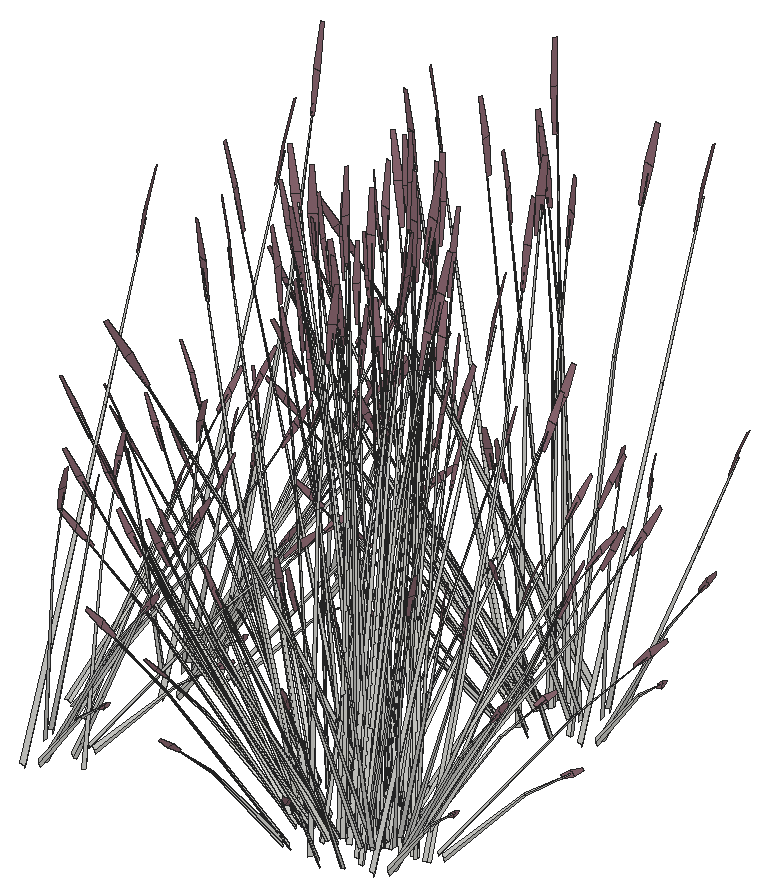
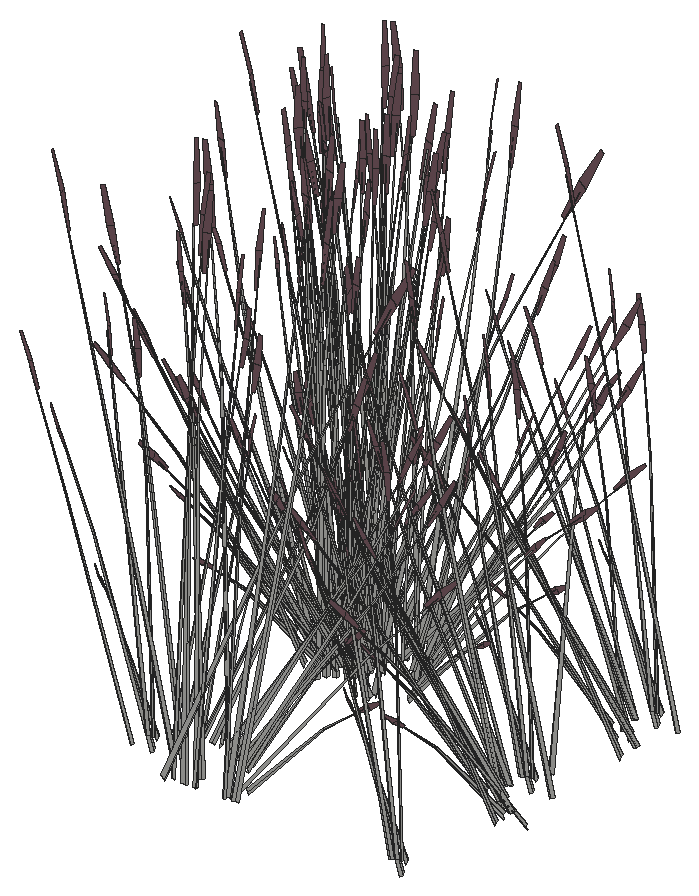
# SketchUp Ruby script. Lengths in inches.
U = 1.inch
M = Sketchup.active_model
def pt(a) = Geom::Point3d.new(a.map { |v| v * U })
def face(e, loops, mat)
  f = e.add_face(loops[0].map { |a| pt(a) })
  loops[1..].each { |l| e.add_face(l.map { |a| pt(a) }).erase! }
  f.material = f.back_material = mat if mat
  f
end
# faces: each face lists its corners as indices into pts; further lists are holes
def faces(e, pts, list, mat = nil) = list.each { |f| face(e, (f[0].is_a?(Array) ? f : [f]).map { |l| l.map { |i| pts[i] } }, mat) }
# xy, xz, yz: faces in a plane at the given z, y or x. An outline is a flat list of corners, or four numbers for a rectangle; further outlines are holes
def ring(l) = l.size == 4 ? [[l[0], l[1]], [l[2], l[1]], [l[2], l[3]], [l[0], l[3]]] : l.each_slice(2).to_a
def flat(e, list, mat, &to3) = list.each { |f| face(e, (f[0].is_a?(Array) ? f : [f]).map { |l| ring(l).map { |u, v| to3.(u, v) } }, mat) }
def xy(e, z, list, mat = nil) = flat(e, list, mat) { |x, y| [x, y, z] }
def xz(e, y, list, mat = nil) = flat(e, list, mat) { |x, z| [x, y, z] }
def yz(e, x, list, mat = nil) = flat(e, list, mat) { |y, z| [x, y, z] }
def lines(e, pts, list) = list.each { |a, b| e.add_line(pt(pts[a]), pt(pts[b])) }
# prism: a flat outline (further loops are holes) pulled along v
def prism(e, loops, v, mat = nil)
  f = face(e, loops, mat); d = Geom::Vector3d.new(v.map { |x| x * U })
  f.pushpull(f.normal.samedirection?(d) ? d.length : -d.length)
end
def box(e, o, s, mat = nil) = prism(e, [[o, [o[0] + s[0], o[1], o[2]], [o[0] + s[0], o[1] + s[1], o[2]], [o[0], o[1] + s[1], o[2]]]], [0, 0, s[2]], mat)
def at(x, y, z, deg = 0) = Geom::Transformation.translation(pt([x, y, z])) * Geom::Transformation.rotation(ORIGIN, Z_AXIS, deg.degrees)
def axes(o, x, y, z) = Geom::Transformation.new([*x, 0, *y, 0, *z, 0, *pt(o).to_a, 1])
def part(name) = M.definitions.add(name)
# library, detail: a bought-in or finely detailed component or shape, given as its bounding box
def library(name, o, s) = part(name).tap { |d| box(d.entities, o, s) }
def detail(e, o, s) = box(e.add_group.entities, o, s)
def put(e, d, t, mat = nil) = e.add_instance(d, t).tap { |i| i.material = mat if mat }
def group(e, t, mat = nil) = e.add_group.tap { |g| g.transformation = t; g.material = mat if mat }.entities
root = M.entities
M.materials.add("LightPink_Translucent").color = [144, 107, 117]
c1 = part("blade")
p = [[2.15,0.21,22],[0,0.17,0],[0.09,0.45,0],[2.18,0.31,22],[2.29,0.31,22],[0.38,0.45,0],
  [2.48,0.24,33],[2.49,0.24,33],[2.48,0.22,33]]
faces(c1.entities,p,[[0,1,2,3],[4,5,2,3],[6,3,4,7],[8,0,3,6]])
c2 = part("seeds")
p = [[0.3,-0.1,1.38],[-0.01,-0.03,1.59],[-0.01,-0.03,0.03],[0.14,-0.07,-0.07],[0.29,-0.03,3],[0.15,0.01,3.11]]
faces(c2.entities,p,[[0,1,2,3],[1,0,4,5]],"LightPink_Translucent")
c3 = part("blade with seeds")
put(c3.entities,c1,at(0,0,0))
put(c3.entities,c2,axes([2.4,0.25,30.99],[1.5799,-0.05474,1.17369],[-0.12525,1.92788,0.29478],[-0.07173,-0.02425,1.56792]))
put(root,c3,axes([34.53,26.82,44.92],[-0.78586,-0.03248,1.0506],[0.51898,-0.68985,0.58006],[0.31045,0.24509,0.8241]))
put(root,c3,axes([35.76,34.52,46.53],[0.82919,-0.54528,-0.35414],[0.78493,0.62262,0.4572],[0.11943,-0.31634,0.87481]))
put(root,c3,axes([35.96,41.53,44.77],[-0.69001,-0.29779,1.1486],[0.89096,-0.30257,0.84392],[0.24031,0.2563,0.25299]))
put(root,c3,axes([33.51,41.21,44.59],[0.02163,-0.34331,1.43002],[1.03345,-0.38348,-0.30754],[0.31903,0.4109,0.61141]))
put(root,c3,axes([38.05,38.59,44.375],[1.53239,0,0],[0,1.1575,-0.51607],[0,0.26363,1.63711]))
put(root,c3,axes([32.86,25.875,46.93],[1.20928,-0.24619,-0.51099],[0.21154,0.93233,-0.3958],[0.32481,0.26718,0.97773]))
put(root,c3,axes([33.97,18.58,44.63],[0.7662,-1.03778,0],[1.28187,0.57875,-0.51607],[0.29196,0.13181,1.63711]))
put(root,c3,axes([36.07,42.88,44.67],[-0.78586,-0.03248,1.0506],[0.51898,-0.68985,0.58006],[0.31045,0.24509,0.8241]))
put(root,c3,axes([35.22,20.32,46.93],[-0.31482,-0.94565,-0.51099],[1.19224,-0.16542,-0.3958],[0.34166,-0.254,0.97773]))
put(root,c3,axes([38.42,21.8,44.51],[-0.75977,-0.66224,-0.06488],[0.83212,-0.6068,-0.29416],[0.23578,-0.04272,0.97024]))
put(root,c3,axes([34.4,41.9375,46.68],[1.20928,-0.24619,-0.51099],[0.21154,0.93233,-0.3958],[0.32481,0.26718,0.97773]))
put(root,c3,axes([36.68,18.43,45.02],[-0.40819,0.5272,1.1486],[-0.35086,-0.70831,0.84392],[0.33713,-0.17749,0.25299]))
put(root,c3,axes([35.51,34.64,44.375],[0.7662,-1.03778,0],[1.28187,0.57875,-0.51607],[0.29196,0.13181,1.63711]))
put(root,c3,axes([36.46,55.41,46.68],[-0.31482,-0.94565,-0.51099],[1.19224,-0.16542,-0.3958],[0.34166,-0.254,0.97773]))
put(root,c3,axes([36.76,36.375,46.68],[-0.31482,-0.94565,-0.51099],[1.19224,-0.16542,-0.3958],[0.34166,-0.254,0.97773]))
put(root,c3,axes([35.25,20.7,47.23],[0.64013,-0.81717,-0.71045],[1.12174,0.58074,0.08574],[0.38221,-0.29607,1.00501]))
put(root,c3,axes([37.93,53.52,44.77],[-0.40819,0.5272,1.1486],[-0.35086,-0.70831,0.84392],[0.33713,-0.17749,0.25299]))
put(root,c3,axes([38.22,34.49,44.77],[-0.40819,0.5272,1.1486],[-0.35086,-0.70831,0.84392],[0.33713,-0.17749,0.25299]))
put(root,c3,axes([37.34,55.5,46.53],[1.06674,-0.14801,-0.35414],[0.28168,0.84611,0.4572],[0.30569,-0.22726,0.87481]))
put(root,c3,axes([36.49,55.79,46.98],[0.64013,-0.81717,-0.71045],[1.12174,0.58074,0.08574],[0.38221,-0.29607,1.00501]))
put(root,c3,axes([37.64,36.48,46.53],[1.06674,-0.14801,-0.35414],[0.28168,0.84611,0.4572],[0.30569,-0.22726,0.87481]))
put(root,c3,axes([35.77,22.42,46.93],[0.332,-0.94205,-0.51099],[1.13828,0.3229,-0.3958],[0.45829,-0.08638,0.97773]))
put(root,c3,axes([36.79,36.76,46.98],[0.64013,-0.81717,-0.71045],[1.12174,0.58074,0.08574],[0.38221,-0.29607,1.00501]))
put(root,c3,axes([38.63,23.02,45.02],[-0.75718,0.17097,1.1486],[0.35641,-0.70661,0.84392],[0.40168,0.04835,0.25299]))
put(root,c3,axes([36.78,41.16,46.53],[0.69728,0.64842,-0.35414],[-0.79619,0.61382,0.4572],[0.40453,0.09339,0.87481]))
put(root,c3,axes([36.17,19.95,44.84],[-0.4378,-0.03068,1.43002],[-0.44851,-0.8229,-0.30754],[0.53783,-0.23279,0.61141]))
put(root,c3,axes([34.5,24.66,47.23],[1.22504,0.02494,-0.71045],[-0.08228,1.05005,0.08574],[0.51899,0.11081,1.00501]))
put(root,c3,axes([36.99,22.68,44.23],[-0.7893,0.12429,1.41583],[-0.12563,-0.9893,0.08104],[0.55282,-0.14974,0.80566]))
put(root,c3,axes([37.3125,38.48,46.68],[0.332,-0.94205,-0.51099],[1.13828,0.3229,-0.3958],[0.45829,-0.08638,0.97773]))
put(root,c3,axes([40.17,39.08,44.77],[-0.75718,0.17097,1.1486],[0.35641,-0.70661,0.84392],[0.40168,0.04835,0.25299]))
put(root,c3,axes([37.42,55.04,44.59],[-0.4378,-0.03068,1.43002],[-0.44851,-0.8229,-0.30754],[0.53783,-0.23279,0.61141]))
put(root,c3,axes([35.55,22.76,47.23],[1.07686,-0.45739,-0.71045],[0.60013,0.94154,0.08574],[0.52031,-0.10696,1.00501]))
put(root,c3,axes([37.72,36.01,44.59],[-0.4378,-0.03068,1.43002],[-0.44851,-0.8229,-0.30754],[0.53783,-0.23279,0.61141]))
put(root,c3,axes([38.01,38.91,46.53],[1.01846,0.28891,-0.35414],[-0.29705,0.84289,0.4572],[0.41005,-0.07729,0.87481]))
put(root,c3,axes([56.85,28.2,44.59],[0.42589,0.08502,1.43002],[0.2745,0.86839,-0.30754],[-0.57851,0.16255,0.61141]))
put(root,c3,axes([36.04,40.72,46.98],[1.22504,0.02494,-0.71045],[-0.08228,1.05005,0.08574],[0.51899,0.11081,1.00501]))
put(root,c3,axes([60.62,25.42,45.34],[0.34834,-0.14982,1.77064],[0.12012,1.04605,0.13857],[-0.75452,0.1388,0.63284]))
put(root,c3,axes([37.21,24.15,44.84],[-0.29514,-0.25472,1.43002],[0.38401,-0.84262,-0.30754],[0.59714,0.11414,0.61141]))
put(root,c3,axes([59.27,51.03,46.98],[-1.22504,-0.02494,-0.71045],[0.08228,-1.05005,0.08574],[-0.51899,-0.11081,1.00501]))
put(root,c3,axes([37.1,38.82,46.98],[1.07686,-0.45739,-0.71045],[0.60013,0.94154,0.08574],[0.52031,-0.10696,1.00501]))
put(root,c3,axes([58.29,51.29,44.59],[0.23927,0.28834,1.43002],[-0.55135,0.78376,-0.30754],[-0.56612,-0.18733,0.61141]))
put(root,c3,axes([59.48,23.75,46.98],[-1.22504,-0.02494,-0.71045],[0.08228,-1.05005,0.08574],[-0.51899,-0.11081,1.00501]))
put(root,c3,axes([58.49,24,44.59],[0.23927,0.28834,1.43002],[-0.55135,0.78376,-0.30754],[-0.56612,-0.18733,0.61141]))
put(root,c3,axes([57.51,25.5625,46.53],[-1.01846,-0.28891,-0.35414],[0.29705,-0.84289,0.4572],[-0.41005,0.07729,0.87481]))
put(root,c3,axes([58.21,25.99,46.68],[-0.332,0.94205,-0.51099],[-1.13828,-0.3229,-0.3958],[-0.45829,0.08638,0.97773]))
put(root,c3,axes([38.75,40.21,44.59],[-0.29514,-0.25472,1.43002],[0.38401,-0.84262,-0.30754],[0.59714,0.11414,0.61141]))
put(root,c3,axes([58.87,51.24,46.68],[-0.88986,0.68603,-0.51099],[-0.77932,-0.72471,-0.3958],[-0.45212,-0.10438,0.97773]))
put(root,c3,axes([59.07,23.96,46.68],[-0.88986,0.68603,-0.51099],[-0.77932,-0.72471,-0.3958],[-0.45212,-0.10438,0.97773]))
put(root,c3,axes([55.96,30.02,44.77],[0.51072,-0.46938,1.1486],[0.20153,0.74307,0.84392],[-0.36908,0.13305,0.25299]))
put(root,c3,axes([58.74,23.3125,46.53],[-0.69728,-0.64842,-0.35414],[0.79619,-0.61382,0.4572],[-0.40453,-0.09339,0.87481]))
put(root,c3,axes([57.89,27.99,46.53],[-1.06674,0.14801,-0.35414],[-0.28168,-0.84611,0.4572],[-0.30569,0.22726,0.87481]))
put(root,c3,axes([56.86,52.15,44.77],[0.78239,-0.07411,1.1486],[-0.49629,0.65296,0.84392],[-0.38663,-0.09795,0.25299]))
put(root,c3,axes([57.07,24.87,44.77],[0.78239,-0.07411,1.1486],[-0.49629,0.65296,0.84392],[-0.38663,-0.09795,0.25299]))
put(root,c3,axes([58.77,28.09,46.68],[0.31482,0.94565,-0.51099],[-1.19224,0.16542,-0.3958],[-0.34166,0.254,0.97773]))
put(root,c3,axes([61.4,49.79,46.98],[-1.04497,-0.50058,-0.71045],[0.74264,-0.8772,0.08574],[-0.3786,-0.29889,1.00501]))
put(root,c3,axes([60.91,49.82,46.68],[-1.20928,0.24619,-0.51099],[-0.21154,-0.93233,-0.3958],[-0.32481,-0.26718,0.97773]))
put(root,c3,axes([61.61,22.51,46.98],[-1.04497,-0.50058,-0.71045],[0.74264,-0.8772,0.08574],[-0.3786,-0.29889,1.00501]))
put(root,c3,axes([61.12,22.53,46.68],[-1.20928,0.24619,-0.51099],[-0.21154,-0.93233,-0.3958],[-0.32481,-0.26718,0.97773]))
put(root,c3,axes([60.76,30.02,44.375],[-0.7662,1.03778,0],[-1.28187,-0.57875,-0.51607],[-0.29196,-0.13181,1.63711]))
put(root,c3,axes([59.37,31.52,44.59],[0.38672,-0.16338,1.43002],[0.95481,0.49262,-0.30754],[-0.28419,0.42626,0.61141]))
put(root,c3,axes([60.23,48.43,44.59],[-0.07421,0.33879,1.43002],[-1.08488,0.28361,-0.30754],[-0.25359,-0.4379,0.61141]))
put(root,c3,axes([60.44,21.14,44.59],[-0.07421,0.33879,1.43002],[-1.08488,0.28361,-0.30754],[-0.25359,-0.4379,0.61141]))
put(root,c3,axes([58.02,53.36,44.375],[-1.53239,0,0],[0,-1.1575,-0.51607],[0,-0.26363,1.63711]))
put(root,c3,axes([61.25,21.84,46.53],[-0.18927,-0.83419,-0.35414],[1.08199,-0.22027,0.4572],[-0.29062,-0.23905,0.87481]))
put(root,c3,axes([58.23,26.07,44.375],[-1.53239,0,0],[0,-1.1575,-0.51607],[0,-0.26363,1.63711]))
put(root,c3,axes([59.76,29.95,46.53],[-0.82919,0.54528,-0.35414],[-0.78493,-0.62262,0.4572],[-0.11943,0.31634,0.87481]))
put(root,c3,axes([59.21,53.05,44.33],[-1.1399,0.87071,0.30756],[-1.1406,-0.86155,-0.36492],[-0.03981,-0.24727,1.64885]))
put(root,c3,axes([63.9,55.46,45.33],[1.05902,0.41762,1.51261],[-1.03748,0.89969,0.59816],[-0.46471,-0.53324,1.26806]))
put(root,c3,axes([59.42,25.76,44.33],[-1.1399,0.87071,0.30756],[-1.1406,-0.86155,-0.36492],[-0.03981,-0.24727,1.64885]))
put(root,c3,axes([59.86,47.88,44.77],[0.63926,0.36046,1.1486],[-0.93099,0.21668,0.84392],[-0.1992,-0.27702,0.25299]))
put(root,c3,axes([64.11,28.17,45.33],[1.05902,0.41762,1.51261],[-1.03748,0.89969,0.59816],[-0.46471,-0.53324,1.26806]))
put(root,c3,axes([60.07,20.6,44.77],[0.63926,0.36046,1.1486],[-0.93099,0.21668,0.84392],[-0.1992,-0.27702,0.25299]))
put(root,c3,axes([60.32,29.375,47.34],[-0.03189,0.95798,-0.7886],[-1.34277,-0.06434,0.09517],[-0.14171,0.40585,1.11556]))
put(root,c3,axes([60.29,32.07,44.77],[-0.03171,-0.6158,1.1486],[0.7925,0.43922,0.84392],[-0.15586,0.29352,0.25299]))
put(root,c3,axes([61.42,29.48,44.48],[1.14694,0.51783,0.49651],[-0.68554,0.92854,0],[-0.26122,-0.11794,1.57504]))
put(root,c3,axes([59.87,30.73,45.36],[0.02693,-0.53464,1.54345],[1.21102,0.2824,0.21329],[-0.10493,0.5698,0.72882]))
put(root,c3,axes([58.95,53.53,44.48],[0,1.03566,0.49651],[-1.37109,0,0],[0,-0.23588,1.57504]))
put(root,c3,axes([63.07,27.87,44.62],[-0.23642,0.92427,0.1448],[-1.15506,-0.16044,-0.41347],[-0.21021,-0.09491,1.26744]))
put(root,c3,axes([59.16,26.25,44.48],[0,1.03566,0.49651],[-1.37109,0,0],[0,-0.23588,1.57504]))
put(root,c3,axes([65.44,30.17,44.19],[-0.75665,-1.04141,-0.05142],[1.28187,-0.57875,0.51607],[-0.31588,0.09915,1.6363]))
put(root,c3,axes([60.59,29.69,47],[0.87728,0.69587,-0.5672],[-0.92674,0.60943,-0.43934],[-0.13348,0.35356,1.08528]))
put(root,c3,axes([65.75,26.17,44.84],[-0.03348,-0.97511,1.41272],[1.51511,0.25277,0.59816],[-0.35835,0.53357,1.3335]))
put(root,c3,axes([63.6,49.39,46.68],[-1.20468,-0.25962,-0.51099],[0.41292,-0.89013,-0.3958],[-0.11046,-0.35838,0.97773]))
put(root,c3,axes([59.64,30.74,44.82],[1.11329,-0.1834,0.06507],[0.25594,0.73887,-0.86304],[-0.07058,0.37403,0.7736]))
put(root,c3,axes([63.81,22.1,46.68],[-1.20468,-0.25962,-0.51099],[0.41292,-0.89013,-0.3958],[-0.11046,-0.35838,0.97773]))
put(root,c3,axes([62.69,26.99,44.36],[1.54892,0.2182,0.45755],[-0.31522,1.23236,0.17955],[-0.22636,-0.119,1.58856]))
put(root,c3,axes([62.08,54.05,44.72],[-0.59459,0.93321,0.44739],[-1.23546,-0.44912,-0.21531],[0,-0.21512,1.43643]))
put(root,c3,axes([64.04,49.55,46.98],[-0.5849,-0.8421,-0.71045],[1.20401,-0.4693,0.08574],[-0.13677,-0.40688,1.00501]))
put(root,c3,axes([62.28,26.77,44.72],[-0.59459,0.93321,0.44739],[-1.23546,-0.44912,-0.21531],[0,-0.21512,1.43643]))
put(root,c3,axes([64.25,22.27,46.98],[-0.5849,-0.8421,-0.71045],[1.20401,-0.4693,0.08574],[-0.13677,-0.40688,1.00501]))
put(root,c3,axes([61.85,28.96,44.47],[1.31687,-0.27488,0.17642],[0.32517,1.02297,0.35086],[-0.11745,-0.14905,1.60407]))
put(root,c3,axes([63.55,29.12,44.2],[-1.23546,-0.46496,0],[0.59459,-0.96613,0],[0,0,1.62707]))
put(root,c3,axes([66.41,30.28,44.375],[0.7662,1.03778,0],[-1.28187,0.57875,-0.51607],[-0.29196,0.13181,1.63711]))
put(root,c3,axes([65.77,29.01,44.47],[0.35402,-1.02926,0.17642],[1.29548,0.29127,0.35086],[-0.22379,0.00501,1.60407]))
put(root,c3,axes([65.17,27.65,44.62],[0.90538,0.62224,0.1448],[-0.75521,0.70202,-0.41347],[-0.21021,0.09491,1.26744]))
put(root,c3,axes([64.85,26.88,44.3],[-1.1399,-0.8914,-0.06131],[1.1406,-0.89194,0],[-0.03981,-0.03113,1.75571]))
put(root,c3,axes([65.15,27.19,44.72],[1.33077,-0.06393,0.44739],[0.12035,1.06125,-0.21531],[-0.23824,0.10756,1.43643]))
put(root,c3,axes([65.48,29.63,44.33],[1.53422,0.33662,0.30756],[-0.38383,1.20322,-0.36492],[-0.25393,0.15059,1.64885]))
put(root,c3,axes([62.34,53.14,44.36],[0.53281,1.15808,0.45755],[-1.52239,0.4027,0.17955],[0.01861,-0.2128,1.58856]))
put(root,c3,axes([66.14,29.56,44.48],[1.14694,-0.51783,0.49651],[0.68554,0.92854,0],[-0.26122,0.11794,1.57504]))
put(root,c3,axes([64.36,21.55,46.53],[0.36946,-0.79643,-0.35414],[1.07787,0.23229,0.4572],[-0.09883,-0.32066,0.87481]))
put(root,c3,axes([62.55,25.85,44.36],[0.53281,1.15808,0.45755],[-1.52239,0.4027,0.17955],[0.01861,-0.2128,1.58856]))
put(root,c3,axes([63.83,28.72,44.2],[-0.39985,-0.89288,0],[1.1418,-0.31268,0],[0,0,1.54371]))
put(root,c3,axes([62.64,30.91,46.53],[-0.36946,0.79643,-0.35414],[-1.07787,-0.23229,0.4572],[0.09883,0.32066,0.87481]))
put(root,c3,axes([64.26,53.24,44.21],[0,-1.19833,0],[1.53239,0,0],[0,0,1.79456]))
put(root,c3,axes([67.79,26.39,44.47],[-0.96285,-0.75439,0.17642],[0.97031,-0.7317,0.35086],[-0.10634,0.15406,1.60407]))
put(root,c3,axes([62.84,53.46,44.43],[1.3808,0.50196,0.24065],[-0.66454,1.04299,0.50002],[0,-0.24043,1.60543]))
put(root,c3,axes([62.39,52.76,44.72],[-1.33077,0.06393,0.44739],[-0.12035,-1.06125,-0.21531],[0.23824,-0.10756,1.43643]))
put(root,c3,axes([64.47,25.95,44.21],[0,-1.19833,0],[1.53239,0,0],[0,0,1.79456]))
put(root,c3,axes([63.04,26.17,44.43],[1.3808,0.50196,0.24065],[-0.66454,1.04299,0.50002],[0,-0.24043,1.60543]))
put(root,c3,axes([65.24,26.43,44.29],[0,1.19774,-0.05637],[-1.53239,0,0],[0,0.03764,1.79368]))
put(root,c3,axes([62.6,25.47,44.72],[-1.33077,0.06393,0.44739],[-0.12035,-1.06125,-0.21531],[0.23824,-0.10756,1.43643]))
put(root,c3,axes([61.98,23.65,44.47],[-0.35402,1.02926,0.17642],[-1.29548,-0.29127,0.35086],[0.22379,-0.00501,1.60407]))
put(root,c3,axes([64.51,28.75,44.29],[0.53281,1.18979,-0.06012],[-1.52239,0.41691,0],[0.01861,0.04155,1.72173]))
put(root,c3,axes([61.14,49.66,44.375],[-0.7662,-1.03778,0],[1.28187,-0.57875,-0.51607],[0.29196,-0.13181,1.63711]))
put(root,c3,axes([61.34,22.38,44.375],[-0.7662,-1.03778,0],[1.28187,-0.57875,-0.51607],[0.29196,-0.13181,1.63711]))
put(root,c3,axes([62.75,30.2,46.98],[0.5849,0.8421,-0.71045],[-1.20401,0.4693,0.08574],[0.13677,0.40688,1.00501]))
put(root,c3,axes([68.91,27.1875,44.2],[-1.53164,-0.00828,-0.04976],[0,-1.1575,0.49943],[-0.04813,0.2635,1.58352]))
put(root,c3,axes([65.9,23.7,44.47],[-1.31687,0.27488,0.17642],[-0.32517,-1.02297,0.35086],[0.11745,0.14905,1.60407]))
put(root,c3,axes([64.34,47.16,44.77],[0.15721,0.60392,1.1486],[-0.87211,-0.33448,0.84392],[0.09385,-0.30923,0.25299]))
put(root,c3,axes([64.55,19.87,44.77],[0.15721,0.60392,1.1486],[-0.87211,-0.33448,0.84392],[0.09385,-0.30923,0.25299]))
put(root,c3,axes([63.74,25.2,44.36],[-1.01611,0.93987,0.45755],[-1.20717,-0.82966,0.17955],[0.24496,-0.0938,1.58856]))
put(root,c3,axes([65.48,26.68,44.21],[0.85545,0.66896,0],[-0.85545,0.66896,0],[0,0,1.69266]))
put(root,c3,axes([65.47,25.9,44.72],[0.59459,-0.93321,0.44739],[1.23546,0.44912,-0.21531],[0,0.21512,1.43643]))
put(root,c3,axes([64.95,29.14,44.2],[1.23546,0.46496,0],[-0.59459,0.96613,0],[0,0,1.74954]))
put(root,c3,axes([63.19,30.37,46.68],[1.20468,0.25962,-0.51099],[-0.41292,0.89013,-0.3958],[0.11046,0.35838,0.97773]))
put(root,c3,axes([65.07,25.67,44.38],[-1.54892,-0.2182,0.49198],[0.31522,-1.23236,0.19306],[0.22636,0.119,1.70813]))
put(root,c3,axes([65.51,26.22,44.21],[1.37109,0,0],[0,1.07219,0],[0,0,1.78407]))
put(root,c3,axes([66.2,50.06,46.68],[-0.87728,-0.69587,-0.51099],[0.92674,-0.60943,-0.3958],[0.13348,-0.35356,0.97773]))
put(root,c3,axes([64.1875,25.04,44.72],[-0.73619,-0.86927,0.44739],[1.11511,-0.61213,-0.21531],[0.23824,0.10756,1.43643]))
put(root,c3,axes([65.98,26.11,44.62],[1.1418,-0.30203,0.1448],[0.39985,0.86246,-0.41347],[0,0.18981,1.26744]))
put(root,c3,axes([66.41,22.77,46.68],[-0.87728,-0.69587,-0.51099],[0.92674,-0.60943,-0.3958],[0.13348,-0.35356,0.97773]))
put(root,c3,axes([65.625,48.83,44.59],[-0.34835,0.20963,1.43002],[-1.04325,-0.36691,-0.30754],[0.19338,-0.4563,0.61141]))
put(root,c3,axes([65.84,21.54,44.59],[-0.34835,0.20963,1.43002],[-1.04325,-0.36691,-0.30754],[0.19338,-0.4563,0.61141]))
put(root,c3,axes([68.59,26.42,44.48],[0,-1.03566,0.49651],[1.37109,0,0],[0,0.23588,1.57504]))
put(root,c3,axes([64.68,24.79,44.62],[0.23642,-0.92427,0.1448],[1.15506,0.16044,-0.41347],[0.21021,0.09491,1.26744]))
put(root,c3,axes([66.12,50.47,44.48],[-1.14694,-0.51783,0.49651],[0.68554,-0.92854,0],[0.26122,0.11794,1.57504]))
put(root,c3,axes([66.47,50.38,46.98],[0.03189,-0.95798,-0.71045],[1.34277,0.06434,0.08574],[0.14171,-0.40585,1.00501]))
put(root,c3,axes([66.33,23.18,44.48],[-1.14694,-0.51783,0.49651],[0.68554,-0.92854,0],[0.26122,0.11794,1.57504]))
put(root,c3,axes([66.68,23.09,46.98],[0.03189,-0.95798,-0.71045],[1.34277,0.06434,0.08574],[0.14171,-0.40585,1.00501]))
put(root,c3,axes([67.24,22.52,46.53],[0.82919,-0.54528,-0.35414],[0.78493,0.62262,0.4572],[0.11943,-0.31634,0.87481]))
put(root,c3,axes([67.43,29.53,44.77],[-0.69001,-0.29779,1.1486],[0.89096,-0.30257,0.84392],[0.24031,0.2563,0.25299]))
put(root,c3,axes([64.98,29.21,44.59],[0.02163,-0.34331,1.43002],[1.03345,-0.38348,-0.30754],[0.31903,0.4109,0.61141]))
put(root,c3,axes([69.52,26.59,44.375],[1.53239,0,0],[0,1.1575,-0.51607],[0,0.26363,1.63711]))
put(root,c3,axes([67.54,30.88,44.67],[-0.78586,-0.03248,1.0506],[0.51898,-0.68985,0.58006],[0.31045,0.24509,0.8241]))
put(root,c3,axes([66.78,49.93,44.375],[0.7662,-1.03778,0],[1.28187,0.57875,-0.51607],[0.29196,0.13181,1.63711]))
put(root,c3,axes([65.875,29.9375,46.68],[1.20928,-0.24619,-0.51099],[0.21154,0.93233,-0.3958],[0.32481,0.26718,0.97773]))
put(root,c3,axes([66.99,22.64,44.375],[0.7662,-1.03778,0],[1.28187,0.57875,-0.51607],[0.29196,0.13181,1.63711]))
put(root,c3,axes([68.02,51.66,46.68],[-0.31482,-0.94565,-0.51099],[1.19224,-0.16542,-0.3958],[0.34166,-0.254,0.97773]))
put(root,c3,axes([68.23,24.375,46.68],[-0.31482,-0.94565,-0.51099],[1.19224,-0.16542,-0.3958],[0.34166,-0.254,0.97773]))
put(root,c3,axes([69.49,49.78,44.77],[-0.40819,0.5272,1.1486],[-0.35086,-0.70831,0.84392],[0.33713,-0.17749,0.25299]))
put(root,c3,axes([69.7,22.49,44.77],[-0.40819,0.5272,1.1486],[-0.35086,-0.70831,0.84392],[0.33713,-0.17749,0.25299]))
put(root,c3,axes([68.06,52.04,46.98],[0.64013,-0.81717,-0.71045],[1.12174,0.58074,0.08574],[0.38221,-0.29607,1.00501]))
put(root,c3,axes([69.11,24.48,46.53],[1.06674,-0.14801,-0.35414],[0.28168,0.84611,0.4572],[0.30569,-0.22726,0.87481]))
put(root,c3,axes([68.26,24.76,46.98],[0.64013,-0.81717,-0.71045],[1.12174,0.58074,0.08574],[0.38221,-0.29607,1.00501]))
put(root,c3,axes([68.25,29.16,46.53],[0.69728,0.64842,-0.35414],[-0.79619,0.61382,0.4572],[0.40453,0.09339,0.87481]))
put(root,c3,axes([68.58,53.76,46.68],[0.332,-0.94205,-0.51099],[1.13828,0.3229,-0.3958],[0.45829,-0.08638,0.97773]))
put(root,c3,axes([68.79,26.48,46.68],[0.332,-0.94205,-0.51099],[1.13828,0.3229,-0.3958],[0.45829,-0.08638,0.97773]))
put(root,c3,axes([71.64,27.08,44.77],[-0.75718,0.17097,1.1486],[0.35641,-0.70661,0.84392],[0.40168,0.04835,0.25299]))
put(root,c3,axes([68.98,51.29,44.59],[-0.4378,-0.03068,1.43002],[-0.44851,-0.8229,-0.30754],[0.53783,-0.23279,0.61141]))
put(root,c3,axes([69.19,24.01,44.59],[-0.4378,-0.03068,1.43002],[-0.44851,-0.8229,-0.30754],[0.53783,-0.23279,0.61141]))
put(root,c3,axes([69.48,26.91,46.53],[1.01846,0.28891,-0.35414],[-0.29705,0.84289,0.4572],[0.41005,-0.07729,0.87481]))
put(root,c3,axes([67.52,28.72,46.98],[1.22504,0.02494,-0.71045],[-0.08228,1.05005,0.08574],[0.51899,0.11081,1.00501]))
put(root,c3,axes([68.57,26.82,46.98],[1.07686,-0.45739,-0.71045],[0.60013,0.94154,0.08574],[0.52031,-0.10696,1.00501]))
put(root,c3,axes([70.23,28.21,44.59],[-0.29514,-0.25472,1.43002],[0.38401,-0.84262,-0.30754],[0.59714,0.11414,0.61141]))
